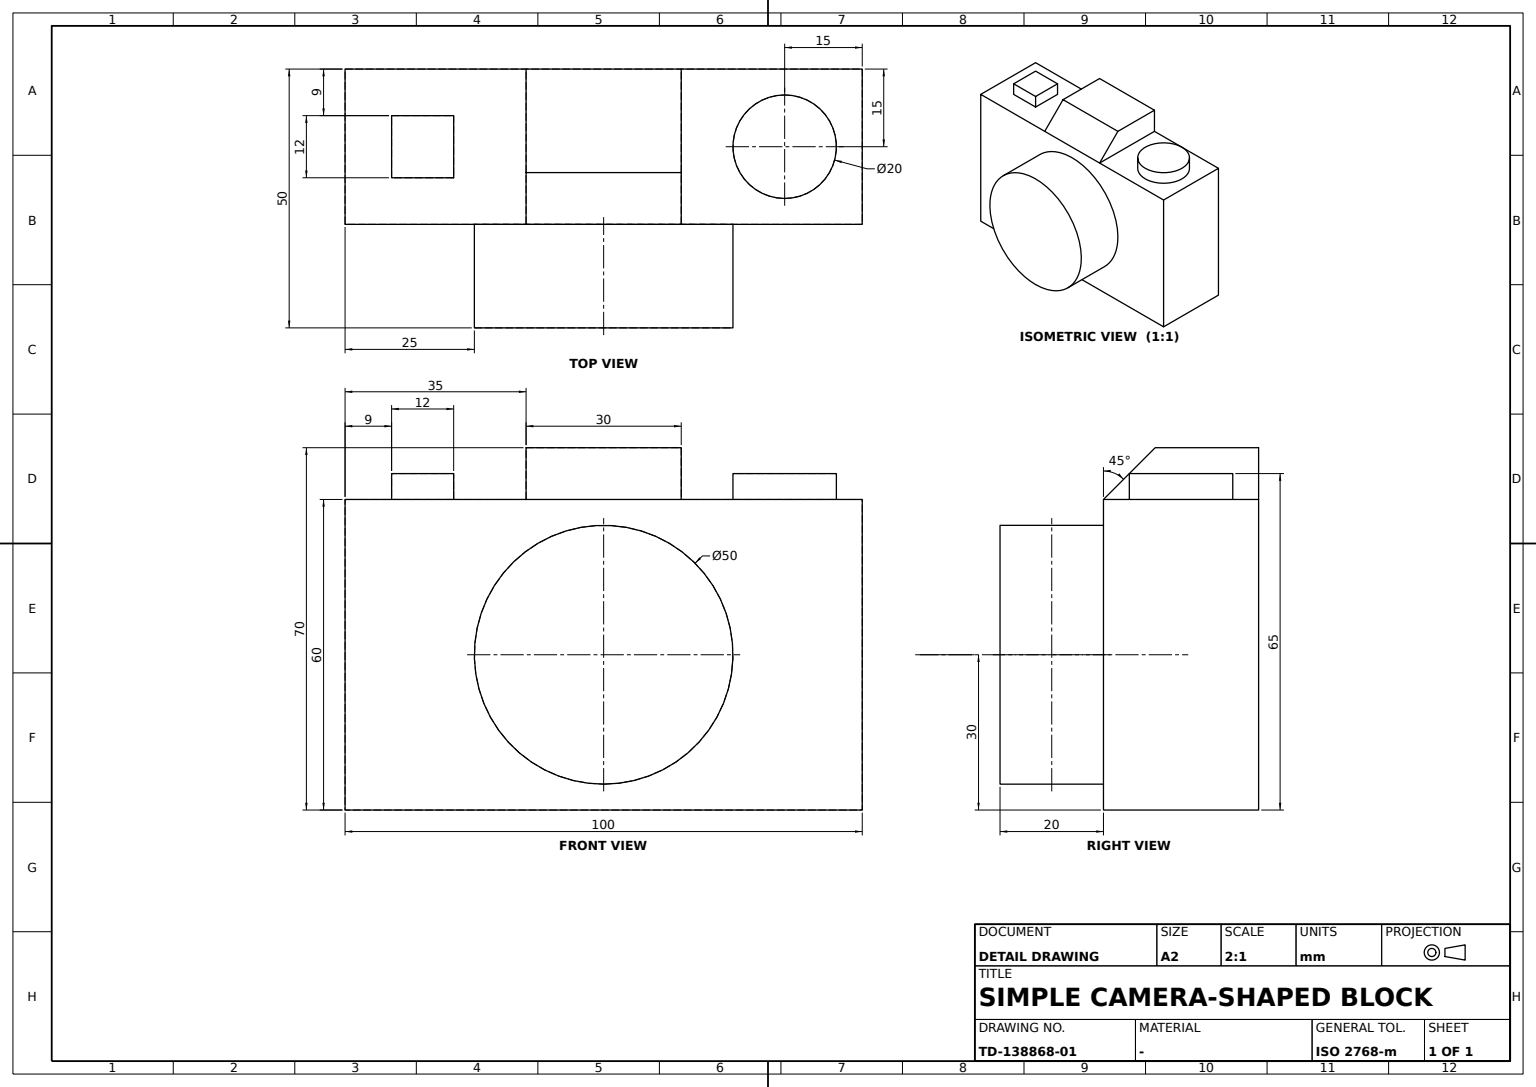
ISO-10303-21;
HEADER;
FILE_DESCRIPTION((''),'2;1');
FILE_NAME('','',(''),(''),'','','');
FILE_SCHEMA(('AUTOMOTIVE_DESIGN'));
ENDSEC;
DATA;
#1=APPLICATION_CONTEXT('');
#2=PRODUCT_CONTEXT('',#1,'mechanical');
#3=PRODUCT('','','',(#2));
#4=PRODUCT_DEFINITION_FORMATION('','',#3);
#5=PRODUCT_DEFINITION_CONTEXT('',#1,'design');
#6=PRODUCT_DEFINITION('','',#4,#5);
#7=PRODUCT_DEFINITION_SHAPE('','',#6);
#8=(LENGTH_UNIT()NAMED_UNIT(*)SI_UNIT(.MILLI.,.METRE.));
#9=(NAMED_UNIT(*)PLANE_ANGLE_UNIT()SI_UNIT($,.RADIAN.));
#10=(NAMED_UNIT(*)SI_UNIT($,.STERADIAN.)SOLID_ANGLE_UNIT());
#11=UNCERTAINTY_MEASURE_WITH_UNIT(LENGTH_MEASURE(0.005),#8,'distance_accuracy_value','');
#12=(GEOMETRIC_REPRESENTATION_CONTEXT(3)GLOBAL_UNCERTAINTY_ASSIGNED_CONTEXT((#11))GLOBAL_UNIT_ASSIGNED_CONTEXT((#8,#9,#10))REPRESENTATION_CONTEXT('',''));
#13=CARTESIAN_POINT('',(6.,-41.,30.));
#14=VERTEX_POINT('',#13);
#15=CARTESIAN_POINT('',(6.,-41.,35.));
#16=VERTEX_POINT('',#15);
#17=DIRECTION('',(0.,0.,1.));
#18=VECTOR('',#17,1000.);
#19=LINE('',#13,#18);
#20=EDGE_CURVE('',#14,#16,#19,.T.);
#21=ORIENTED_EDGE('',*,*,#20,.F.);
#22=CARTESIAN_POINT('',(6.,-29.,30.));
#23=VERTEX_POINT('',#22);
#24=DIRECTION('',(0.,-1.,0.));
#25=VECTOR('',#24,1000.);
#26=LINE('',#22,#25);
#27=EDGE_CURVE('',#23,#14,#26,.T.);
#28=ORIENTED_EDGE('',*,*,#27,.F.);
#29=CARTESIAN_POINT('',(6.,-29.,35.));
#30=VERTEX_POINT('',#29);
#31=LINE('',#22,#18);
#32=EDGE_CURVE('',#23,#30,#31,.T.);
#33=ORIENTED_EDGE('',*,*,#32,.T.);
#34=CARTESIAN_POINT('',(6.,0.,35.));
#35=LINE('',#34,#25);
#36=EDGE_CURVE('',#30,#16,#35,.T.);
#37=ORIENTED_EDGE('',*,*,#36,.T.);
#38=EDGE_LOOP('',(#21,#28,#33,#37));
#39=FACE_BOUND('',#38,.T.);
#40=DIRECTION('',(-1.,0.,0.));
#41=AXIS2_PLACEMENT_3D('',#22,#40,#24);
#42=PLANE('',#41);
#43=ADVANCED_FACE('',(#39),#42,.F.);
#44=CARTESIAN_POINT('',(-10.,35.,30.));
#45=VERTEX_POINT('',#44);
#46=CARTESIAN_POINT('',(0.,35.,30.));
#47=DIRECTION('',(0.,0.,-1.));
#48=AXIS2_PLACEMENT_3D('',#46,#47,#40);
#49=CIRCLE('',#48,10.);
#50=EDGE_CURVE('',#45,#45,#49,.F.);
#51=ORIENTED_EDGE('',*,*,#50,.T.);
#52=EDGE_LOOP('',(#51));
#53=FACE_BOUND('',#52,.T.);
#54=CARTESIAN_POINT('',(10.,35.,35.));
#55=VERTEX_POINT('',#54);
#56=CARTESIAN_POINT('',(0.,35.,35.));
#57=DIRECTION('',(1.,0.,0.));
#58=AXIS2_PLACEMENT_3D('',#56,#17,#57);
#59=CIRCLE('',#58,10.);
#60=EDGE_CURVE('',#55,#55,#59,.T.);
#61=ORIENTED_EDGE('',*,*,#60,.F.);
#62=EDGE_LOOP('',(#61));
#63=FACE_BOUND('',#62,.T.);
#64=CARTESIAN_POINT('',(0.,35.,32.5));
#65=DIRECTION('',(0.,1.,0.));
#66=AXIS2_PLACEMENT_3D('',#64,#17,#65);
#67=CYLINDRICAL_SURFACE('',#66,10.);
#68=ADVANCED_FACE('',(#53,#63),#67,.T.);
#69=CARTESIAN_POINT('',(-15.,-15.,40.));
#70=VERTEX_POINT('',#69);
#71=CARTESIAN_POINT('',(-15.,15.,40.));
#72=VERTEX_POINT('',#71);
#73=CARTESIAN_POINT('',(-15.,0.,40.));
#74=VECTOR('',#65,1000.);
#75=LINE('',#73,#74);
#76=EDGE_CURVE('',#70,#72,#75,.T.);
#77=ORIENTED_EDGE('',*,*,#76,.F.);
#78=CARTESIAN_POINT('',(5.,-15.,40.));
#79=VERTEX_POINT('',#78);
#80=CARTESIAN_POINT('',(0.,-15.,40.));
#81=VECTOR('',#57,1000.);
#82=LINE('',#80,#81);
#83=EDGE_CURVE('',#70,#79,#82,.T.);
#84=ORIENTED_EDGE('',*,*,#83,.T.);
#85=CARTESIAN_POINT('',(5.,15.,40.));
#86=VERTEX_POINT('',#85);
#87=CARTESIAN_POINT('',(5.,0.,40.));
#88=LINE('',#87,#74);
#89=EDGE_CURVE('',#79,#86,#88,.T.);
#90=ORIENTED_EDGE('',*,*,#89,.T.);
#91=CARTESIAN_POINT('',(0.,15.,40.));
#92=LINE('',#91,#81);
#93=EDGE_CURVE('',#72,#86,#92,.T.);
#94=ORIENTED_EDGE('',*,*,#93,.F.);
#95=EDGE_LOOP('',(#77,#84,#90,#94));
#96=FACE_BOUND('',#95,.T.);
#97=AXIS2_PLACEMENT_3D('',#73,#17,#57);
#98=PLANE('',#97);
#99=ADVANCED_FACE('',(#96),#98,.T.);
#100=ORIENTED_EDGE('',*,*,#36,.F.);
#101=CARTESIAN_POINT('',(-6.,-29.,35.));
#102=VERTEX_POINT('',#101);
#103=CARTESIAN_POINT('',(0.,-29.,35.));
#104=LINE('',#103,#81);
#105=EDGE_CURVE('',#102,#30,#104,.T.);
#106=ORIENTED_EDGE('',*,*,#105,.F.);
#107=CARTESIAN_POINT('',(-6.,-41.,35.));
#108=VERTEX_POINT('',#107);
#109=CARTESIAN_POINT('',(-6.,0.,35.));
#110=LINE('',#109,#74);
#111=EDGE_CURVE('',#108,#102,#110,.T.);
#112=ORIENTED_EDGE('',*,*,#111,.F.);
#113=CARTESIAN_POINT('',(0.,-41.,35.));
#114=VECTOR('',#40,1000.);
#115=LINE('',#113,#114);
#116=EDGE_CURVE('',#16,#108,#115,.T.);
#117=ORIENTED_EDGE('',*,*,#116,.F.);
#118=EDGE_LOOP('',(#100,#106,#112,#117));
#119=FACE_BOUND('',#118,.T.);
#120=CARTESIAN_POINT('',(0.,0.,35.));
#121=AXIS2_PLACEMENT_3D('',#120,#17,#65);
#122=PLANE('',#121);
#123=ADVANCED_FACE('',(#119),#122,.T.);
#124=CARTESIAN_POINT('',(-6.,-29.,30.));
#125=VERTEX_POINT('',#124);
#126=LINE('',#124,#81);
#127=EDGE_CURVE('',#125,#23,#126,.T.);
#128=ORIENTED_EDGE('',*,*,#127,.F.);
#129=LINE('',#124,#18);
#130=EDGE_CURVE('',#125,#102,#129,.T.);
#131=ORIENTED_EDGE('',*,*,#130,.T.);
#132=ORIENTED_EDGE('',*,*,#105,.T.);
#133=ORIENTED_EDGE('',*,*,#32,.F.);
#134=EDGE_LOOP('',(#128,#131,#132,#133));
#135=FACE_BOUND('',#134,.T.);
#136=AXIS2_PLACEMENT_3D('',#124,#24,#57);
#137=PLANE('',#136);
#138=ADVANCED_FACE('',(#135),#137,.F.);
#139=ORIENTED_EDGE('',*,*,#116,.T.);
#140=CARTESIAN_POINT('',(-6.,-41.,30.));
#141=VERTEX_POINT('',#140);
#142=LINE('',#140,#18);
#143=EDGE_CURVE('',#141,#108,#142,.T.);
#144=ORIENTED_EDGE('',*,*,#143,.F.);
#145=LINE('',#13,#114);
#146=EDGE_CURVE('',#14,#141,#145,.T.);
#147=ORIENTED_EDGE('',*,*,#146,.F.);
#148=ORIENTED_EDGE('',*,*,#20,.T.);
#149=EDGE_LOOP('',(#139,#144,#147,#148));
#150=FACE_BOUND('',#149,.T.);
#151=AXIS2_PLACEMENT_3D('',#13,#65,#40);
#152=PLANE('',#151);
#153=ADVANCED_FACE('',(#150),#152,.F.);
#154=CARTESIAN_POINT('',(15.,-50.,30.));
#155=VERTEX_POINT('',#154);
#156=CARTESIAN_POINT('',(15.,-15.,30.));
#157=VERTEX_POINT('',#156);
#158=CARTESIAN_POINT('',(15.,0.,30.));
#159=LINE('',#158,#74);
#160=EDGE_CURVE('',#155,#157,#159,.T.);
#161=ORIENTED_EDGE('',*,*,#160,.T.);
#162=CARTESIAN_POINT('',(-15.,-15.,30.));
#163=VERTEX_POINT('',#162);
#164=CARTESIAN_POINT('',(0.,-15.,30.));
#165=LINE('',#164,#114);
#166=EDGE_CURVE('',#157,#163,#165,.T.);
#167=ORIENTED_EDGE('',*,*,#166,.T.);
#168=CARTESIAN_POINT('',(-15.,-50.,30.));
#169=VERTEX_POINT('',#168);
#170=CARTESIAN_POINT('',(-15.,0.,30.));
#171=LINE('',#170,#74);
#172=EDGE_CURVE('',#169,#163,#171,.T.);
#173=ORIENTED_EDGE('',*,*,#172,.F.);
#174=CARTESIAN_POINT('',(0.,-50.,30.));
#175=LINE('',#174,#81);
#176=EDGE_CURVE('',#169,#155,#175,.T.);
#177=ORIENTED_EDGE('',*,*,#176,.T.);
#178=EDGE_LOOP('',(#161,#167,#173,#177));
#179=FACE_BOUND('',#178,.T.);
#180=LINE('',#140,#74);
#181=EDGE_CURVE('',#141,#125,#180,.T.);
#182=ORIENTED_EDGE('',*,*,#181,.T.);
#183=ORIENTED_EDGE('',*,*,#127,.T.);
#184=ORIENTED_EDGE('',*,*,#27,.T.);
#185=ORIENTED_EDGE('',*,*,#146,.T.);
#186=EDGE_LOOP('',(#182,#183,#184,#185));
#187=FACE_BOUND('',#186,.T.);
#188=AXIS2_PLACEMENT_3D('',#174,#47,#65);
#189=PLANE('',#188);
#190=ADVANCED_FACE('',(#179,#187),#189,.F.);
#191=ORIENTED_EDGE('',*,*,#166,.F.);
#192=CARTESIAN_POINT('',(22.5,-15.,22.5));
#193=DIRECTION('',(0.707106781,0.,-0.707106781));
#194=VECTOR('',#193,1000.);
#195=LINE('',#192,#194);
#196=EDGE_CURVE('',#79,#157,#195,.T.);
#197=ORIENTED_EDGE('',*,*,#196,.F.);
#198=ORIENTED_EDGE('',*,*,#83,.F.);
#199=CARTESIAN_POINT('',(-15.,-15.,0.));
#200=LINE('',#199,#18);
#201=EDGE_CURVE('',#163,#70,#200,.T.);
#202=ORIENTED_EDGE('',*,*,#201,.F.);
#203=EDGE_LOOP('',(#191,#197,#198,#202));
#204=FACE_BOUND('',#203,.T.);
#205=CARTESIAN_POINT('',(0.,-15.,0.));
#206=AXIS2_PLACEMENT_3D('',#205,#65,#40);
#207=PLANE('',#206);
#208=ADVANCED_FACE('',(#204),#207,.F.);
#209=ORIENTED_EDGE('',*,*,#60,.T.);
#210=EDGE_LOOP('',(#209));
#211=FACE_BOUND('',#210,.T.);
#212=ADVANCED_FACE('',(#211),#122,.T.);
#213=CARTESIAN_POINT('',(-15.,15.,30.));
#214=VERTEX_POINT('',#213);
#215=CARTESIAN_POINT('',(-15.,15.,0.));
#216=LINE('',#215,#18);
#217=EDGE_CURVE('',#214,#72,#216,.T.);
#218=ORIENTED_EDGE('',*,*,#217,.T.);
#219=ORIENTED_EDGE('',*,*,#93,.T.);
#220=CARTESIAN_POINT('',(15.,15.,30.));
#221=VERTEX_POINT('',#220);
#222=CARTESIAN_POINT('',(22.5,15.,22.5));
#223=LINE('',#222,#194);
#224=EDGE_CURVE('',#86,#221,#223,.T.);
#225=ORIENTED_EDGE('',*,*,#224,.T.);
#226=CARTESIAN_POINT('',(0.,15.,30.));
#227=LINE('',#226,#114);
#228=EDGE_CURVE('',#221,#214,#227,.T.);
#229=ORIENTED_EDGE('',*,*,#228,.T.);
#230=EDGE_LOOP('',(#218,#219,#225,#229));
#231=FACE_BOUND('',#230,.T.);
#232=CARTESIAN_POINT('',(0.,15.,0.));
#233=AXIS2_PLACEMENT_3D('',#232,#65,#40);
#234=PLANE('',#233);
#235=ADVANCED_FACE('',(#231),#234,.T.);
#236=CARTESIAN_POINT('',(-15.,50.,-30.));
#237=VERTEX_POINT('',#236);
#238=CARTESIAN_POINT('',(-15.,-50.,-30.));
#239=VERTEX_POINT('',#238);
#240=CARTESIAN_POINT('',(-15.,0.,-30.));
#241=LINE('',#240,#25);
#242=EDGE_CURVE('',#237,#239,#241,.T.);
#243=ORIENTED_EDGE('',*,*,#242,.T.);
#244=CARTESIAN_POINT('',(-15.,-50.,0.));
#245=LINE('',#244,#18);
#246=EDGE_CURVE('',#239,#169,#245,.T.);
#247=ORIENTED_EDGE('',*,*,#246,.T.);
#248=ORIENTED_EDGE('',*,*,#172,.T.);
#249=ORIENTED_EDGE('',*,*,#201,.T.);
#250=ORIENTED_EDGE('',*,*,#76,.T.);
#251=ORIENTED_EDGE('',*,*,#217,.F.);
#252=CARTESIAN_POINT('',(-15.,50.,30.));
#253=VERTEX_POINT('',#252);
#254=EDGE_CURVE('',#214,#253,#171,.T.);
#255=ORIENTED_EDGE('',*,*,#254,.T.);
#256=CARTESIAN_POINT('',(-15.,50.,0.));
#257=VECTOR('',#47,1000.);
#258=LINE('',#256,#257);
#259=EDGE_CURVE('',#253,#237,#258,.T.);
#260=ORIENTED_EDGE('',*,*,#259,.T.);
#261=EDGE_LOOP('',(#243,#247,#248,#249,#250,#251,#255,#260));
#262=FACE_BOUND('',#261,.T.);
#263=CARTESIAN_POINT('',(-15.,0.,0.));
#264=AXIS2_PLACEMENT_3D('',#263,#57,#65);
#265=PLANE('',#264);
#266=ADVANCED_FACE('',(#262),#265,.F.);
#267=ORIENTED_EDGE('',*,*,#143,.T.);
#268=ORIENTED_EDGE('',*,*,#111,.T.);
#269=ORIENTED_EDGE('',*,*,#130,.F.);
#270=ORIENTED_EDGE('',*,*,#181,.F.);
#271=EDGE_LOOP('',(#267,#268,#269,#270));
#272=FACE_BOUND('',#271,.T.);
#273=AXIS2_PLACEMENT_3D('',#140,#57,#65);
#274=PLANE('',#273);
#275=ADVANCED_FACE('',(#272),#274,.F.);
#276=CARTESIAN_POINT('',(15.,50.,-30.));
#277=VERTEX_POINT('',#276);
#278=CARTESIAN_POINT('',(0.,50.,-30.));
#279=LINE('',#278,#81);
#280=EDGE_CURVE('',#237,#277,#279,.T.);
#281=ORIENTED_EDGE('',*,*,#280,.T.);
#282=CARTESIAN_POINT('',(15.,-50.,-30.));
#283=VERTEX_POINT('',#282);
#284=CARTESIAN_POINT('',(15.,0.,-30.));
#285=LINE('',#284,#25);
#286=EDGE_CURVE('',#277,#283,#285,.T.);
#287=ORIENTED_EDGE('',*,*,#286,.T.);
#288=CARTESIAN_POINT('',(0.,-50.,-30.));
#289=LINE('',#288,#81);
#290=EDGE_CURVE('',#239,#283,#289,.T.);
#291=ORIENTED_EDGE('',*,*,#290,.F.);
#292=ORIENTED_EDGE('',*,*,#242,.F.);
#293=EDGE_LOOP('',(#281,#287,#291,#292));
#294=FACE_BOUND('',#293,.T.);
#295=AXIS2_PLACEMENT_3D('',#278,#17,#24);
#296=PLANE('',#295);
#297=ADVANCED_FACE('',(#294),#296,.F.);
#298=CARTESIAN_POINT('',(15.,50.,30.));
#299=VERTEX_POINT('',#298);
#300=EDGE_CURVE('',#221,#299,#159,.T.);
#301=ORIENTED_EDGE('',*,*,#300,.T.);
#302=CARTESIAN_POINT('',(0.,50.,30.));
#303=LINE('',#302,#81);
#304=EDGE_CURVE('',#253,#299,#303,.T.);
#305=ORIENTED_EDGE('',*,*,#304,.F.);
#306=ORIENTED_EDGE('',*,*,#254,.F.);
#307=ORIENTED_EDGE('',*,*,#228,.F.);
#308=EDGE_LOOP('',(#301,#305,#306,#307));
#309=FACE_BOUND('',#308,.T.);
#310=ORIENTED_EDGE('',*,*,#50,.F.);
#311=EDGE_LOOP('',(#310));
#312=FACE_BOUND('',#311,.T.);
#313=ADVANCED_FACE('',(#309,#312),#189,.F.);
#314=CARTESIAN_POINT('',(35.,0.,-25.));
#315=VERTEX_POINT('',#314);
#316=CARTESIAN_POINT('',(35.,0.,0.));
#317=AXIS2_PLACEMENT_3D('',#316,#57,#47);
#318=CIRCLE('',#317,25.);
#319=EDGE_CURVE('',#315,#315,#318,.T.);
#320=ORIENTED_EDGE('',*,*,#319,.F.);
#321=EDGE_LOOP('',(#320));
#322=FACE_BOUND('',#321,.T.);
#323=CARTESIAN_POINT('',(15.,0.,-25.));
#324=VERTEX_POINT('',#323);
#325=CARTESIAN_POINT('',(15.,0.,0.));
#326=AXIS2_PLACEMENT_3D('',#325,#57,#47);
#327=CIRCLE('',#326,25.);
#328=EDGE_CURVE('',#324,#324,#327,.T.);
#329=ORIENTED_EDGE('',*,*,#328,.T.);
#330=EDGE_LOOP('',(#329));
#331=FACE_BOUND('',#330,.T.);
#332=CARTESIAN_POINT('',(25.,0.,0.));
#333=AXIS2_PLACEMENT_3D('',#332,#57,#65);
#334=CYLINDRICAL_SURFACE('',#333,25.);
#335=ADVANCED_FACE('',(#322,#331),#334,.T.);
#336=ORIENTED_EDGE('',*,*,#280,.F.);
#337=ORIENTED_EDGE('',*,*,#259,.F.);
#338=ORIENTED_EDGE('',*,*,#304,.T.);
#339=CARTESIAN_POINT('',(15.,50.,0.));
#340=LINE('',#339,#257);
#341=EDGE_CURVE('',#299,#277,#340,.T.);
#342=ORIENTED_EDGE('',*,*,#341,.T.);
#343=EDGE_LOOP('',(#336,#337,#338,#342));
#344=FACE_BOUND('',#343,.T.);
#345=AXIS2_PLACEMENT_3D('',#302,#24,#47);
#346=PLANE('',#345);
#347=ADVANCED_FACE('',(#344),#346,.F.);
#348=ORIENTED_EDGE('',*,*,#319,.T.);
#349=EDGE_LOOP('',(#348));
#350=FACE_BOUND('',#349,.T.);
#351=AXIS2_PLACEMENT_3D('',#316,#57,#65);
#352=PLANE('',#351);
#353=ADVANCED_FACE('',(#350),#352,.T.);
#354=ORIENTED_EDGE('',*,*,#290,.T.);
#355=CARTESIAN_POINT('',(15.,-50.,0.));
#356=LINE('',#355,#18);
#357=EDGE_CURVE('',#283,#155,#356,.T.);
#358=ORIENTED_EDGE('',*,*,#357,.T.);
#359=ORIENTED_EDGE('',*,*,#176,.F.);
#360=ORIENTED_EDGE('',*,*,#246,.F.);
#361=EDGE_LOOP('',(#354,#358,#359,#360));
#362=FACE_BOUND('',#361,.T.);
#363=AXIS2_PLACEMENT_3D('',#288,#65,#17);
#364=PLANE('',#363);
#365=ADVANCED_FACE('',(#362),#364,.F.);
#366=ORIENTED_EDGE('',*,*,#196,.T.);
#367=EDGE_CURVE('',#157,#221,#159,.T.);
#368=ORIENTED_EDGE('',*,*,#367,.T.);
#369=ORIENTED_EDGE('',*,*,#224,.F.);
#370=ORIENTED_EDGE('',*,*,#89,.F.);
#371=EDGE_LOOP('',(#366,#368,#369,#370));
#372=FACE_BOUND('',#371,.T.);
#373=DIRECTION('',(0.707106781,0.,0.707106781));
#374=AXIS2_PLACEMENT_3D('',#87,#373,#193);
#375=PLANE('',#374);
#376=ADVANCED_FACE('',(#372),#375,.T.);
#377=ORIENTED_EDGE('',*,*,#328,.F.);
#378=EDGE_LOOP('',(#377));
#379=FACE_BOUND('',#378,.T.);
#380=ORIENTED_EDGE('',*,*,#160,.F.);
#381=ORIENTED_EDGE('',*,*,#357,.F.);
#382=ORIENTED_EDGE('',*,*,#286,.F.);
#383=ORIENTED_EDGE('',*,*,#341,.F.);
#384=ORIENTED_EDGE('',*,*,#300,.F.);
#385=ORIENTED_EDGE('',*,*,#367,.F.);
#386=EDGE_LOOP('',(#380,#381,#382,#383,#384,#385));
#387=FACE_BOUND('',#386,.T.);
#388=AXIS2_PLACEMENT_3D('',#325,#57,#65);
#389=PLANE('',#388);
#390=ADVANCED_FACE('',(#379,#387),#389,.T.);
#391=CLOSED_SHELL('',(#43,#68,#99,#123,#138,#153,#190,#208,#212,#235,#266,#275,#297,#313,#335,#347,#353,#365,#376,#390));
#392=MANIFOLD_SOLID_BREP('',#391);
#393=ADVANCED_BREP_SHAPE_REPRESENTATION('',(#392),#12);
#394=SHAPE_DEFINITION_REPRESENTATION(#7,#393);
ENDSEC;
END-ISO-10303-21;
